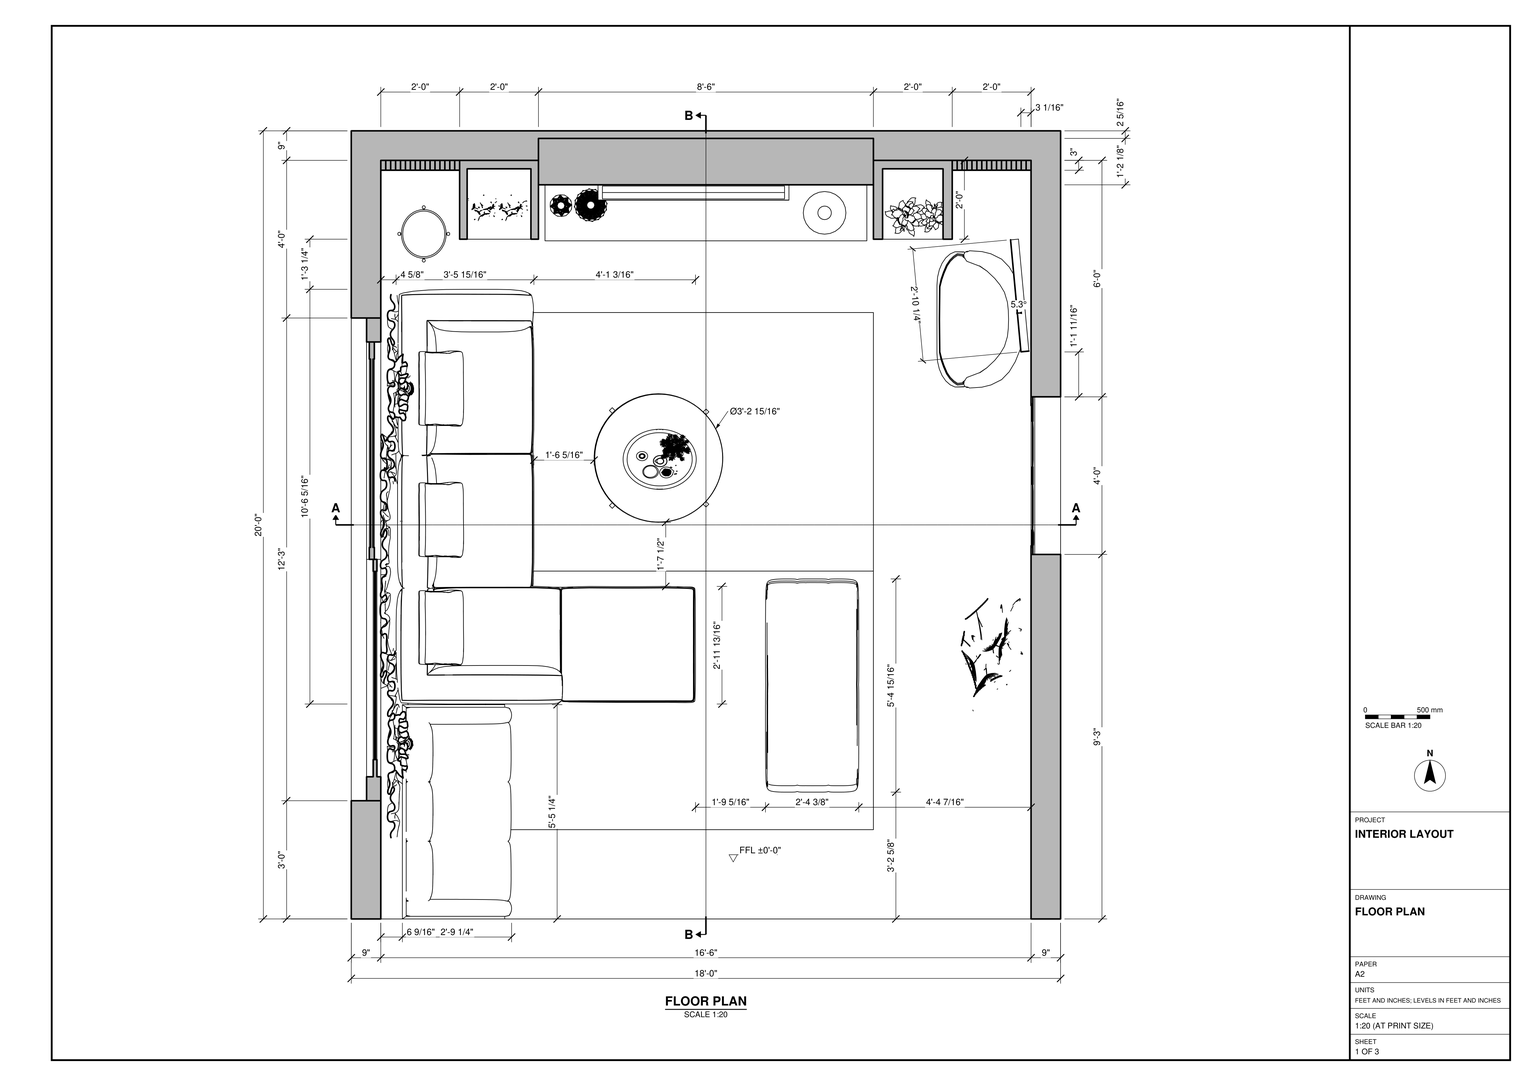
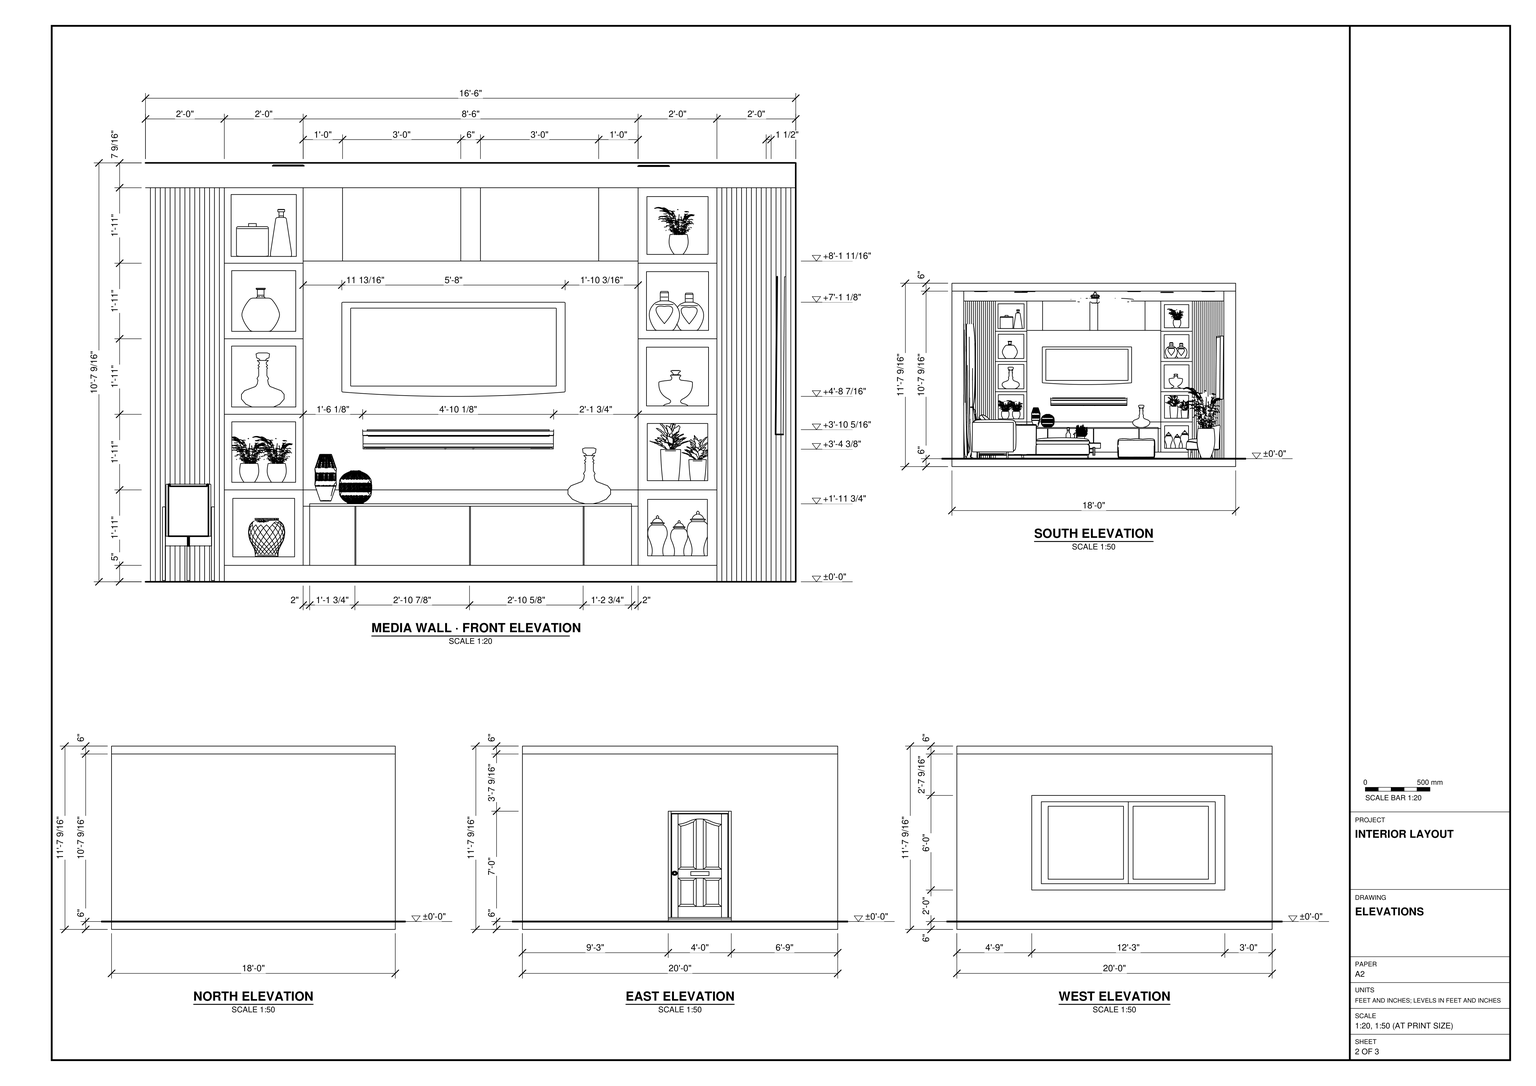
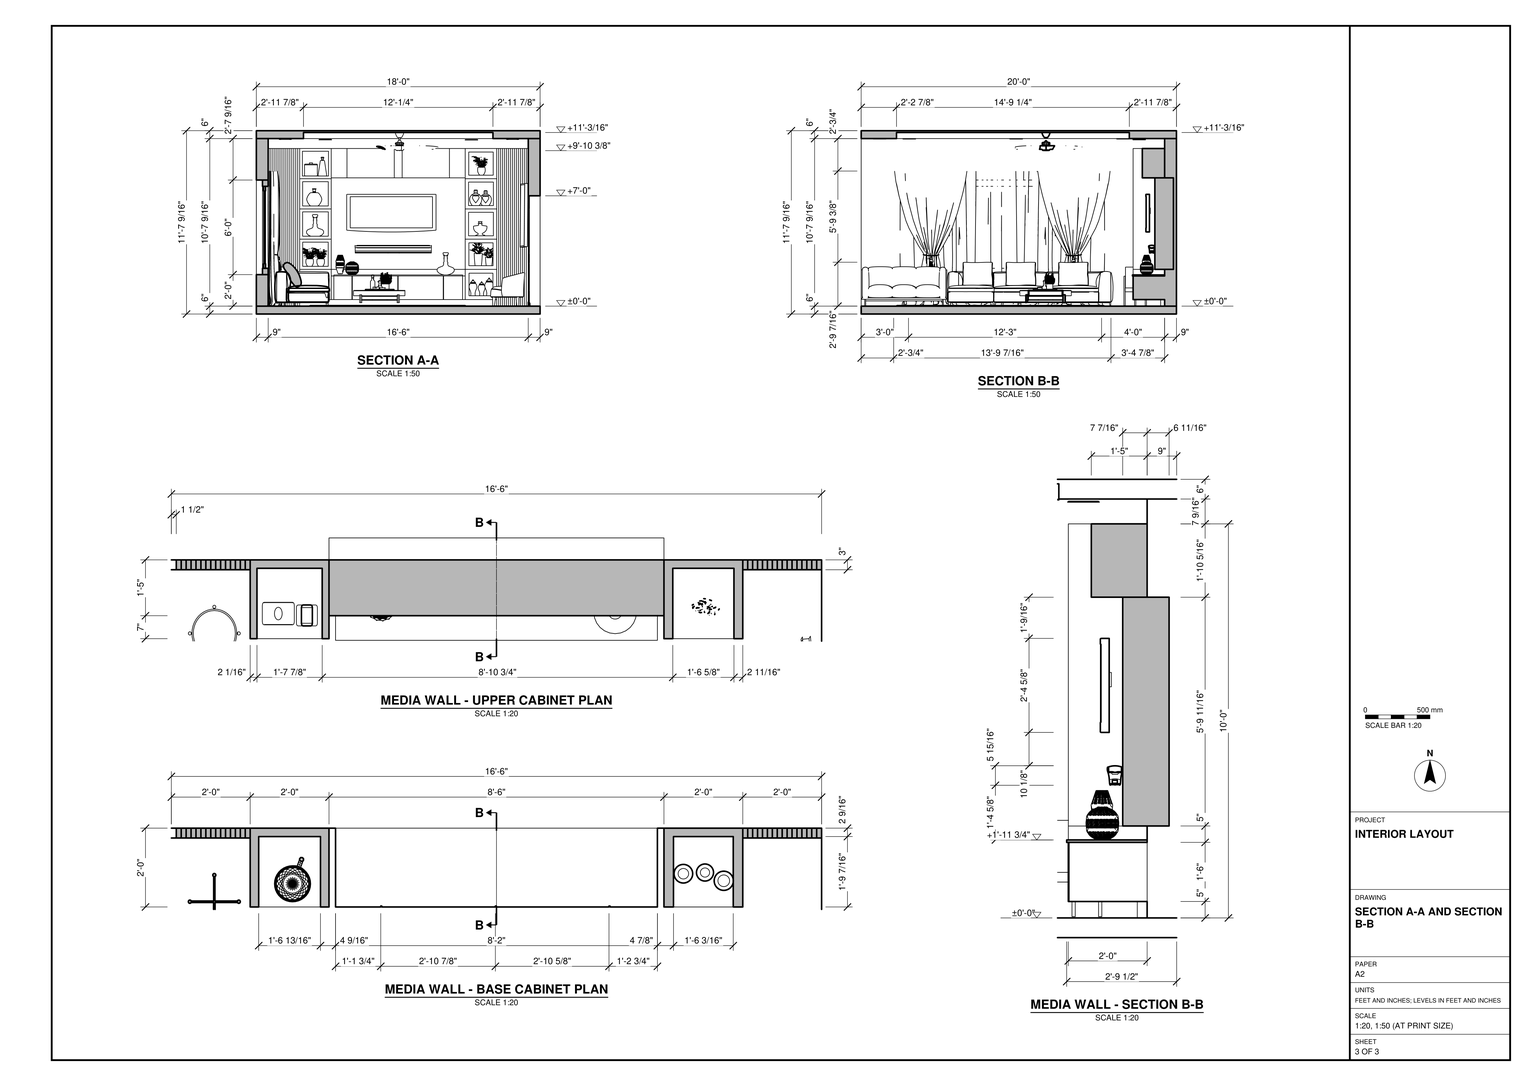
Build the living room in SketchUp from task_files/diagram_01.pdf. Work in feet and inches. The room measures 18'-0" east to west by 20'-0" north to south, with an overall height of 11'-7 9/16". Use ±0'-0" as the finished floor level. Model the 9" walls on the north, east and west sides, leaving the south side open as shown. Include the floor and roof slabs, the stepped ceiling, the framed window and curtains on the west wall, and the door in the east wall.

Fit the media joinery across the north wall. Use the front elevation for the cabinet divisions and shelf spacing, and the cabinet plans and section for the depths, plinth and projections. Place the screen and horizontal speaker between the base and upper cabinets. Flank this bay with open display shelves and finish the outer ends with vertical slats.

Arrange the sectional sofa along the window wall with its chaise extending into the room. Place the round coffee table beside the sectional, the long ottoman east of the chaise, the separate seat at the southwest end and the armchair near the northeast corner. Include the rug beneath the seating area, the ceiling fan and the display objects in the positions shown. Decor and loose items may be any suitable library components, for example from 3D Warehouse.

Keep the walls, slabs and roof, and each furniture or joinery piece, in separate groups or components. Use components for repeated parts. Save one SketchUp model as output_files/furnished_living_room_with_a_built_in_media_wall.skp.

# SketchUp Ruby script. Lengths in inches.
U = 1.inch
M = Sketchup.active_model
def pt(a) = Geom::Point3d.new(a.map { |v| v * U })
def face(e, loops, mat)
  f = e.add_face(loops[0].map { |a| pt(a) })
  loops[1..].each { |l| e.add_face(l.map { |a| pt(a) }).erase! }
  f.material = f.back_material = mat if mat
  f
end
# faces: each face lists its corners as indices into pts; further lists are holes
def faces(e, pts, list, mat = nil) = list.each { |f| face(e, (f[0].is_a?(Array) ? f : [f]).map { |l| l.map { |i| pts[i] } }, mat) }
# xy, xz, yz: faces in a plane at the given z, y or x. An outline is a flat list of corners, or four numbers for a rectangle; further outlines are holes
def ring(l) = l.size == 4 ? [[l[0], l[1]], [l[2], l[1]], [l[2], l[3]], [l[0], l[3]]] : l.each_slice(2).to_a
def flat(e, list, mat, &to3) = list.each { |f| face(e, (f[0].is_a?(Array) ? f : [f]).map { |l| ring(l).map { |u, v| to3.(u, v) } }, mat) }
def xy(e, z, list, mat = nil) = flat(e, list, mat) { |x, y| [x, y, z] }
def xz(e, y, list, mat = nil) = flat(e, list, mat) { |x, z| [x, y, z] }
def yz(e, x, list, mat = nil) = flat(e, list, mat) { |y, z| [x, y, z] }
def lines(e, pts, list) = list.each { |a, b| e.add_line(pt(pts[a]), pt(pts[b])) }
# prism: a flat outline (further loops are holes) pulled along v
def prism(e, loops, v, mat = nil)
  f = face(e, loops, mat); d = Geom::Vector3d.new(v.map { |x| x * U })
  f.pushpull(f.normal.samedirection?(d) ? d.length : -d.length)
end
def box(e, o, s, mat = nil) = prism(e, [[o, [o[0] + s[0], o[1], o[2]], [o[0] + s[0], o[1] + s[1], o[2]], [o[0], o[1] + s[1], o[2]]]], [0, 0, s[2]], mat)
def at(x, y, z, deg = 0) = Geom::Transformation.translation(pt([x, y, z])) * Geom::Transformation.rotation(ORIGIN, Z_AXIS, deg.degrees)
def axes(o, x, y, z) = Geom::Transformation.new([*x, 0, *y, 0, *z, 0, *pt(o).to_a, 1])
def part(name) = M.definitions.add(name)
# library, detail: a bought-in or finely detailed component or shape, given as its bounding box
def library(name, o, s) = part(name).tap { |d| box(d.entities, o, s) }
def detail(e, o, s) = box(e.add_group.entities, o, s)
def put(e, d, t, mat = nil) = e.add_instance(d, t).tap { |i| i.material = mat if mat }
def group(e, t, mat = nil) = e.add_group.tap { |g| g.transformation = t; g.material = mat if mat }.entities
root = M.entities
M.materials.add("CANDLELIGHT BEIGE UC96693").color = [242, 236, 220]
M.materials.add("Translucide ambre1").color = [255, 156, 130]
M.materials["Translucide ambre1"].alpha = 0.5
M.materials.add("Transparence  25").color = [255, 255, 255]
M.materials.add("[Carrera Marble]").color = [207, 207, 207]
M.materials.add("[Color D01]").color = [255, 240, 188]
M.materials.add("[Color D02]").color = [255, 229, 153]
M.materials.add("[Color M08]1").color = [30, 30, 30]
M.materials.add("[Formica Beige]").color = [211, 187, 149]
M.materials.add("[Quartz Light Brown]").color = [242, 230, 205]
M.materials.add("[Translucent_Glass_Safety]").color = [204, 235, 244]
M.materials["[Translucent_Glass_Safety]"].alpha = 0.5
M.materials.add("[Translucent_Glass_Sky_Reflection]").color = [125, 138, 183]
M.materials["[Translucent_Glass_Sky_Reflection]"].alpha = 0.52
M.materials.add("[Wood Bamboo]").color = [198, 132, 75]
M.materials.add("[Wood Floor Light]").color = [204, 176, 127]
M.materials.add("z1").color = [147, 146, 137]
c1 = part("Sliding window")
xy(c1.entities,0,[[0,0,4.33,55.51]])
xy(c1.entities,2.76,[[0,2.76,2,27.76],[3.15,2.76,4.33,27.76],[0,27.76,0.82,52.76],[0.82,27.76,2.36,52.76],[2.36,27.76,4.33,52.76]])
xy(c1.entities,4.72,[[2,4.72,2.4,26.38],[2.76,4.72,3.15,26.38],[0.82,29.13,1.22,50.79],[1.97,29.13,2.36,50.79]])
xy(c1.entities,36.61,[[2,4.72,2.4,26.38],[2.76,4.72,3.15,26.38],[0.82,29.13,1.22,50.79],[1.97,29.13,2.36,50.79]])
xy(c1.entities,38.58,[[0,2.76,2,27.76],[3.15,2.76,4.33,27.76],[0,27.76,0.82,52.76],[0.82,27.76,2.36,52.76],[2.36,27.76,4.33,52.76]])
xy(c1.entities,41.34,[[0,0,4.33,55.51]])
xz(c1.entities,0,[[0,0,4.33,41.34]])
xz(c1.entities,2.76,[[0,2.76,2,38.58],[3.15,2.76,4.33,38.58]])
xz(c1.entities,4.72,[[2,4.72,2.4,36.61],[2.76,4.72,3.15,36.61]])
xz(c1.entities,26.38,[[2,4.72,2.4,36.61],[2.76,4.72,3.15,36.61]])
xz(c1.entities,27.76,[[0.82,2.76,2,38.58],[2,2.76,2.36,38.58],[2.36,2.76,3.15,38.58]])
xz(c1.entities,29.13,[[0.82,4.72,1.22,36.61],[1.97,4.72,2.36,36.61]])
xz(c1.entities,50.79,[[0.82,4.72,1.22,36.61],[1.97,4.72,2.36,36.61]])
xz(c1.entities,52.76,[[0,2.76,0.82,38.58],[0.82,2.76,2.36,38.58],[2.36,2.76,4.33,38.58]])
xz(c1.entities,55.51,[[0,0,4.33,41.34]])
yz(c1.entities,0,[[[0,0,55.51,41.34],[2.76,2.76,52.76,38.58]]])
yz(c1.entities,0.82,[[[27.76,2.76,52.76,38.58],[29.13,4.72,50.79,36.61]]])
yz(c1.entities,1.22,[[29.13,4.72,50.79,36.61]],"[Translucent_Glass_Sky_Reflection]")
yz(c1.entities,1.97,[[29.13,4.72,50.79,36.61]],"[Translucent_Glass_Sky_Reflection]")
yz(c1.entities,2,[[[2.76,2.76,27.76,38.58],[4.72,4.72,26.38,36.61]]])
yz(c1.entities,2.36,[[[27.76,2.76,52.76,38.58],[29.13,4.72,50.79,36.61]]])
yz(c1.entities,2.4,[[4.72,4.72,26.38,36.61]],"[Translucent_Glass_Safety]")
yz(c1.entities,2.76,[[4.72,4.72,26.38,36.61]],"[Translucent_Glass_Safety]")
yz(c1.entities,3.15,[[[2.76,2.76,27.76,38.58],[4.72,4.72,26.38,36.61]]])
yz(c1.entities,4.33,[[[0,0,55.51,41.34],[2.76,2.76,52.76,38.58]]])
c2 = library("door2",[0,0,0],[35.42,7.875,78.74])
c3 = library("michel-club1",[-34.67,-0.85,-0.13],[126.28,91.17,33.41])
c4 = library("BANK+STOEL+MET+RONDE+LEUNING",[-13.09,-13.32,0],[26.18,25.9,25.63])
c5 = library("25984",[-0.01,-37.35,0],[37.87,32.46,16.84])
c6 = part("DDR842RVS01100X")
xy(c6.entities,0,[[-70.87,0,47.24,78.74]])
xy(c6.entities,0.39,[[-70.87,0,47.24,78.74]],"[Quartz Light Brown]")
xz(c6.entities,0,[[-70.87,0,47.24,0.39]])
xz(c6.entities,78.74,[[-70.87,0,47.24,0.39]])
yz(c6.entities,-70.87,[[0,0,78.74,0.39]])
yz(c6.entities,47.24,[[0,0,78.74,0.39]])
c7 = library("Potted plant",[1.65,0,0],[13.63,13.63,20.73])
c8 = library("Group3\#1",[-238.15,54.18,0],[46.4,43.96,56.68])
c9 = library("Untitled",[82.71,28.87,-11.8125],[39.77,1.97,25.2])
c10 = library("Wisdom Sage Series P38m ( On Wall )",[6.24,4.69,38.8125],[7.11,5.95,34.2])
c11 = library("Plant+pots+03",[-13.35,-27.09,0],[26.22,40.73,41.57])
c12 = library("Light+01",[-2.3,-2.42,-0.19],[4.85,4.84,0.19])
c13 = library("Avation+Styled+Ceiling+Fan_JSB",[-19.77,-29.63,-13.8125],[51.59,58.16,13.8125])
c14 = library("Group\#2",[0,0,0],[10.53,165.43,102.59])
c15 = part("Group\#3")
xy(c15.entities,120,[[0,0,1.5,3]])
xz(c15.entities,0,[[0,0,1.5,120]])
yz(c15.entities,1.5,[[0,5,3,120]])
c16 = library("Group\#5",[0,0,0],[112.99,39.26,34.22])
c17 = library("Group\#11",[0,0,0],[33.52,33.48,12.25])
c18 = part("Groupe\#39")
xy(c18.entities,0.1,[[0.39,0.3125,3.55,1.07]],"Translucide ambre1")
xy(c18.entities,3.46,[[0.2,0,3.75,0,3.85,0.03,3.92,0.1,3.94,0.2,3.94,1.18,3.92,1.28,3.85,1.35,3.75,1.38,0.2,1.38,0.1,1.35,0.03,1.28,0,1.18,0,0.2,0.03,0.1,0.1,0.03]])
xz(c18.entities,0,[[0.2,0.2,3.75,3.46]],"Translucide ambre1")
xz(c18.entities,1.38,[[0.2,0.2,3.75,3.46]],"Translucide ambre1")
yz(c18.entities,0,[[0.2,0.2,1.18,3.46]],"Translucide ambre1")
yz(c18.entities,3.94,[[0.2,0.2,1.18,3.46]],"Translucide ambre1")
p = [[0.15,0.11,0.03],[0.11,0.05,0.1],[0.05,0.11,0.1],[0.11,0.15,0.03],[0.2,0.1,0.03],[0.2,0.03,0.1],
  [3.75,0.1,0.03],[3.75,0.03,0.1],[3.8,0.11,0.03],[3.83,0.05,0.1],[3.83,0.15,0.03],[3.9,0.11,0.1],
  [0.03,0.2,0.1],[0.1,0.2,0.03],[0.2,0.2,0],[3.75,0.2,0],[3.85,0.2,0.03],[3.92,0.2,0.1],
  [0.1,1.18,0.03],[0.03,1.18,0.1],[0.2,1.18,0],[0.39,1.07,0.1],[0.39,0.3125,0.1],[3.55,0.3125,0.1],
  [3.55,1.07,0.1],[3.75,1.18,0],[3.85,1.18,0.03],[3.92,1.18,0.1],[0.11,1.33,0.1],[0.15,1.27,0.03],
  [0.11,1.23,0.03],[0.05,1.27,0.1],[0.2,1.28,0.03],[3.75,1.28,0.03],[3.83,1.23,0.03],[3.8,1.27,0.03],
  [3.9,1.27,0.1],[3.83,1.33,0.1],[0.2,1.35,0.1],[3.75,1.35,0.1],[0.1,0.03,0.2],[0.03,0.1,0.2],
  [0.2,0,0.2],[3.75,0,0.2],[3.85,0.03,0.2],[3.92,0.1,0.2],[0,0.2,0.2],[3.94,0.2,0.2],
  [0,1.18,0.2],[3.94,1.18,0.2],[0.03,1.28,0.2],[3.92,1.28,0.2],[0.1,1.35,0.2],[0.2,1.38,0.2],
  [3.75,1.38,0.2],[3.85,1.35,0.2],[0.1,0.03,3.46],[0.03,0.1,3.46],[0.2,0,3.46],[3.75,0,3.46],
  [3.85,0.03,3.46],[3.92,0.1,3.46],[0,0.2,3.46],[3.94,0.2,3.46],[0.03,1.28,3.46],[0,1.18,3.46],
  [3.92,1.28,3.46],[3.94,1.18,3.46],[0.1,1.35,3.46],[3.85,1.35,3.46],[0.2,1.38,3.46],[3.75,1.38,3.46]]
faces(c18.entities,p,[[0,1,2,3],[4,5,1,0],[4,6,7,5],[7,6,8,9],[9,8,10,11],[3,2,12,13],[14,0,3],[14,3,13],
  [14,4,0],[14,15,6,4],[8,15,10],[10,15,16],[6,15,8],[11,10,16,17],[18,13,12,19],[20,14,13,18],
  [20,21,22,14],[14,22,23,15],[24,25,15,23],[15,25,26,16],[16,26,27,17],[25,24,21,20],[28,29,30,31],[31,30,18,19],
  [29,20,30],[30,20,18],[32,20,29],[25,20,32,33],[25,34,26],[25,33,35],[25,35,34],[34,36,27,26],
  [35,37,36,34],[38,32,29,28],[33,32,38,39],[33,39,37,35],[1,40,41,2],[5,42,40,1],[5,7,43,42],[43,7,9,44],
  [44,9,11,45],[2,41,46,12],[45,11,17,47],[19,12,46,48],[17,27,49,47],[50,31,19,48],[36,51,49,27],[52,28,31,50],
  [53,38,28,52],[39,54,55,37],[37,55,51,36],[39,38,53,54],[40,56,57,41],[42,58,56,40],[59,43,44,60],[60,44,45,61],
  [41,57,62,46],[61,45,47,63],[64,50,48,65],[51,66,67,49],[68,52,50,64],[55,69,66,51],[70,53,52,68],[54,71,69,55]],"Translucide ambre1")
c19 = part("Groupe\#53")
prism(c19.entities,[[[0,0.47,0],[0,0.53,0],[0.01,0.59,0],[0.03,0.65,0],[0.06,0.7,0],[0.09,0.75,0],[0.13,0.8,0],[0.17,0.84,0],[0.22,0.87,0],[0.27,0.9,0],[0.33,0.92,0],[0.38,0.9375,0],[0.44,0.95,0],[0.5,0.95,0],[0.5625,0.9375,0],[0.62,0.92,0],[0.68,0.9,0],[0.73,0.87,0],[0.78,0.84,0],[0.82,0.8,0],[0.86,0.75,0],[0.89,0.7,0],[0.91,0.65,0],[0.93,0.59,0],[0.94,0.53,0],[0.95,0.47,0],[0.94,0.41,0],[0.93,0.35,0],[0.91,0.3,0],[0.89,0.24,0],[0.86,0.19,0],[0.82,0.15,0],[0.78,0.11,0],[0.73,0.07,0],[0.68,0.04,0],[0.62,0.02,0],[0.5625,0.01,0],[0.5,0,0],[0.44,0,0],[0.38,0.01,0],[0.33,0.02,0],[0.27,0.04,0],[0.22,0.07,0],[0.17,0.11,0],[0.13,0.15,0],[0.09,0.19,0],[0.06,0.24,0],[0.03,0.3,0],[0.01,0.35,0],[0,0.41,0]]],[0,0,0.38])
c20 = part("Groupe\#24")
xy(c20.entities,0.1,[[0.39,0.3125,3.55,1.07]])
xy(c20.entities,3.66,[[0.2,0.2,3.75,1.18]])
xz(c20.entities,0,[[[0.2,0.2,3.75,3.46],[0.8125,0.8125,3.13,2.85]]])
xz(c20.entities,0,[[0.8125,0.8125,3.13,2.85]],"CANDLELIGHT BEIGE UC96693")
xz(c20.entities,1.38,[[0.2,0.2,3.75,3.46]])
yz(c20.entities,0,[[0.2,0.2,1.18,3.46]])
yz(c20.entities,3.94,[[0.2,0.2,1.18,3.46]])
p = [[0.15,0.11,0.03],[0.11,0.05,0.1],[0.05,0.11,0.1],[0.11,0.15,0.03],[0.2,0.1,0.03],[0.2,0.03,0.1],
  [3.75,0.1,0.03],[3.75,0.03,0.1],[3.8,0.11,0.03],[3.83,0.05,0.1],[3.83,0.15,0.03],[3.9,0.11,0.1],
  [0.03,0.2,0.1],[0.1,0.2,0.03],[0.2,0.2,0],[3.75,0.2,0],[3.85,0.2,0.03],[3.92,0.2,0.1],
  [0.1,1.18,0.03],[0.03,1.18,0.1],[0.2,1.18,0],[0.39,1.07,0.1],[0.39,0.3125,0.1],[3.55,0.3125,0.1],
  [3.55,1.07,0.1],[3.75,1.18,0],[3.85,1.18,0.03],[3.92,1.18,0.1],[0.11,1.33,0.1],[0.15,1.27,0.03],
  [0.11,1.23,0.03],[0.05,1.27,0.1],[0.2,1.28,0.03],[3.75,1.28,0.03],[3.83,1.23,0.03],[3.8,1.27,0.03],
  [3.9,1.27,0.1],[3.83,1.33,0.1],[0.2,1.35,0.1],[3.75,1.35,0.1],[0.1,0.03,0.2],[0.03,0.1,0.2],
  [0.2,0,0.2],[3.75,0,0.2],[3.85,0.03,0.2],[3.92,0.1,0.2],[0,0.2,0.2],[3.94,0.2,0.2],
  [0,1.18,0.2],[3.94,1.18,0.2],[0.03,1.28,0.2],[3.92,1.28,0.2],[0.1,1.35,0.2],[0.2,1.38,0.2],
  [3.75,1.38,0.2],[3.85,1.35,0.2],[0.1,0.03,3.46],[0.03,0.1,3.46],[0.2,0,3.46],[3.75,0,3.46],
  [3.85,0.03,3.46],[3.92,0.1,3.46],[0,0.2,3.46],[3.94,0.2,3.46],[0.03,1.28,3.46],[0,1.18,3.46],
  [3.92,1.28,3.46],[3.94,1.18,3.46],[0.1,1.35,3.46],[3.85,1.35,3.46],[0.2,1.38,3.46],[3.75,1.38,3.46],
  [0.11,0.05,3.5625],[0.05,0.11,3.5625],[0.2,0.03,3.5625],[3.75,0.03,3.5625],[3.83,0.05,3.5625],[3.9,0.11,3.5625],
  [0.03,0.2,3.5625],[3.92,0.2,3.5625],[0.03,1.18,3.5625],[3.92,1.18,3.5625],[0.05,1.27,3.5625],[3.9,1.27,3.5625],
  [0.11,1.33,3.5625],[0.2,1.35,3.5625],[3.75,1.35,3.5625],[3.83,1.33,3.5625],[0.15,0.11,3.64],[0.11,0.15,3.64],
  [0.2,0.1,3.64],[3.75,0.1,3.64],[3.8,0.11,3.64],[3.83,0.15,3.64],[0.1,0.2,3.64],[0.2,0.2,3.66],
  [3.75,0.2,3.66],[3.85,0.2,3.64],[0.1,1.18,3.64],[0.2,1.18,3.66],[3.75,1.18,3.66],[3.85,1.18,3.64],
  [0.15,1.27,3.64],[0.11,1.23,3.64],[0.2,1.28,3.64],[3.75,1.28,3.64],[3.8,1.27,3.64],[3.83,1.23,3.64]]
faces(c20.entities,p,[[0,1,2,3],[4,5,1,0],[4,6,7,5],[7,6,8,9],[9,8,10,11],[3,2,12,13],[14,0,3],[14,3,13],
  [14,4,0],[14,15,6,4],[8,15,10],[10,15,16],[6,15,8],[11,10,16,17],[18,13,12,19],[20,14,13,18],
  [20,21,22,14],[14,22,23,15],[24,25,15,23],[15,25,26,16],[16,26,27,17],[25,24,21,20],[28,29,30,31],[31,30,18,19],
  [29,20,30],[30,20,18],[32,20,29],[25,20,32,33],[25,34,26],[25,33,35],[25,35,34],[34,36,27,26],
  [35,37,36,34],[38,32,29,28],[33,32,38,39],[33,39,37,35],[1,40,41,2],[5,42,40,1],[5,7,43,42],[43,7,9,44],
  [44,9,11,45],[2,41,46,12],[45,11,17,47],[19,12,46,48],[17,27,49,47],[50,31,19,48],[36,51,49,27],[52,28,31,50],
  [53,38,28,52],[39,54,55,37],[37,55,51,36],[39,38,53,54],[40,56,57,41],[42,58,56,40],[59,43,44,60],[60,44,45,61],
  [41,57,62,46],[61,45,47,63],[64,50,48,65],[51,66,67,49],[68,52,50,64],[55,69,66,51],[70,53,52,68],[54,71,69,55],
  [56,72,73,57],[58,74,72,56],[75,74,58,59],[75,59,60,76],[76,60,61,77],[57,73,78,62],[77,61,63,79],[78,80,65,62],
  [81,79,63,67],[82,64,65,80],[66,83,81,67],[84,68,64,82],[85,70,68,84],[71,86,87,69],[69,87,83,66],[85,86,71,70],
  [72,88,89,73],[74,90,88,72],[91,90,74,75],[91,75,76,92],[92,76,77,93],[73,89,94,78],[90,95,88],[88,95,89],
  [89,95,94],[96,95,90,91],[96,91,92],[96,92,93],[96,93,97],[93,77,79,97],[94,98,80,78],[95,99,98,94],
  [100,96,97,101],[101,97,79,81],[102,84,82,103],[103,82,80,98],[99,104,102],[99,102,103],[99,103,98],[99,100,105,104],
  [105,100,106],[106,100,107],[107,100,101],[83,107,101,81],[87,106,107,83],[104,85,84,102],[104,105,86,85],[86,105,106,87]])
c21 = part("Groupe\#77")
put(c21.entities,c19,at(1.5,0.375,3.66),"Transparence  25")
put(c21.entities,c20,axes([0,0,0],[1,0,0],[0,1.23,0],[0,0,1]),"Transparence  25")
c22 = part("Groupe\#128")
put(c22.entities,c18,axes([0.06,0.03,0.05],[0.97,0,0],[0,1.1931,0],[0,0,0.97]),"Translucide ambre1")
put(c22.entities,c21,at(0,0,0))
c23 = library("Group\#20",[0,0,0],[4.2,4.19,4.43])
c24 = library("Group\#21",[0,0,0],[3.96,1.38,4.54])
c25 = library("Group\#24",[0,0,0],[2.58,1.57,5.86])
c26 = library("Group\#25",[0,0,0],[159.9,159.9,209.38])
c27 = library("Group\#30",[0,0,0],[2.89,0.98,3.73])
c28 = library("Group\#203",[0,0,0],[42.29,73.125,63.36])
c29 = library("Group\#213",[0,0,0],[12.8,10.5625,11.04])
c30 = library("Group\#33",[0,0,0],[16.42,7.45,12.07])
c31 = library("Group\#48",[0,0,0],[18.31,18.31,13.72])
xy(root,-6,[[0,0,216,240]],"[Color D02]")
xy(root,0,[[9,0,207,0,207,111,216,111,216,159,207,159,207,231,184.5,231,184.5,228,183,228,183,231,9,231]],"[Color D01]")
xy(root,0,[[0,0,9,0,9,231,207,231,207,159,216,159,216,240,0,240],[207,0,216,111],[183,228,184.5,231]],"[Color D02]")
xy(root,5,[[33,207,57,231],[59,207,59,231,157,231,157,207,142.5625,207,142.5625,207.3,142.26,207.3,142.26,207,107.96,207,107.96,207.3,107.66,207.3,107.66,207,73.0625,207,73.0625,207.3,72.76,207.3,72.76,207],[159,207,183,231]],"[Color D02]")
xy(root,7.59,[[35.59,207,54.41,228.4375]],"[Wood Bamboo]")
xy(root,7.9,[[161.9,207,180.1,228.4375]],"[Wood Bamboo]")
xy(root,23,[[59,206.5,72.76,207],[72.76,206.5,73.0625,207.3],[73.0625,206.5,107.66,207],[107.66,206.5,107.96,207.3],[107.96,206.5,142.26,207],
  [142.26,206.5,142.5625,207.3],[142.5625,206.5,157,207],[59,207,59,231,157,231,157,207,142.5625,207,142.5625,207.3,142.26,207.3,142.26,207,107.96,207,107.96,207.3,107.66,207.3,107.66,207,73.0625,207,73.0625,207.3,72.76,207.3,72.76,207]],"[Color D02]")
xy(root,23.75,[[59,206.5,157,231]],"[Wood Bamboo]")
xy(root,24,[[0,36,9,183]],"[Color D02]")
xy(root,25.1,[[161.9,207,180.1,228.4375]],"[Wood Bamboo]")
xy(root,25.41,[[35.59,207,54.41,228.4375]],"[Wood Bamboo]")
xy(root,28,[[57,223.5625,159,231],[57,231,159,237.6875]],"[Color D02]")
xy(root,30.29,[[35.29,207,54.71,228.4375]],"[Wood Bamboo]")
xy(root,30.79,[[161.79,207,180.21,228.4375]],"[Wood Bamboo]")
xy(root,48.21,[[161.79,207,180.21,228.4375]],"[Wood Bamboo]")
xy(root,48.71,[[35.29,207,54.71,228.4375]])
xy(root,53.23,[[35.23,207,54.77,228.4375]],"[Wood Bamboo]")
xy(root,53.55,[[161.55,207,180.45,228.4375]],"[Wood Bamboo]")
xy(root,71.45,[[161.55,207,180.45,228.4375]],"[Wood Bamboo]")
xy(root,71.77,[[35.23,207,54.77,228.4375]],"[Wood Bamboo]")
xy(root,76.25,[[35.25,207,54.75,228.4375]],"[Wood Bamboo]")
xy(root,76.55,[[161.55,207,180.45,228.4375]],"[Wood Bamboo]")
xy(root,84,[[207,111,216,159]],"[Color D02]")
xy(root,94.45,[[161.55,207,180.45,228.4375]],"[Wood Bamboo]")
xy(root,94.75,[[35.25,207,54.75,228.4375]],"[Wood Bamboo]")
xy(root,96,[[0,36,9,183]],"[Color D02]")
xy(root,97.67,[[57,214,159,223.5625],[57,223.5625,159,231],[57,231,159,237.6875]],"[Color D02]")
xy(root,99.07,[[35.07,207,54.93,228.4375]],"[Wood Bamboo]")
xy(root,99.6875,[[161.6875,207,180.3125,228.4375]],"[Wood Bamboo]")
xy(root,117.3125,[[161.6875,207,180.3125,228.4375]],"[Wood Bamboo]")
xy(root,117.93,[[35.07,207,54.93,228.4375]],"[Wood Bamboo]")
xy(root,120,[[57,214,159,231]],"[Color D01]")
xy(root,120,[[33,207,57,231],[159,207,183,231]],"[Wood Bamboo]")
xy(root,127.5625,[[0,0,0,240,216,240,216,0,207,0,207,231,9,231,9,0],[[9,0,207,231],[35.89,26.89,180.11,204.11]]],"[Color D01]")
xy(root,132.1875,[[35.89,26.89,180.11,204.11]],"[Color D01]")
xy(root,133.5625,[[0,0,216,240]])
xz(root,0,[[0,127.5625,216,133.5625]])
xz(root,0,[[0,0,9,127.5625],[207,0,216,127.5625]],"[Color D01]")
xz(root,0,[[0,-6,216,0]],"[Color D02]")
xz(root,26.89,[[35.89,127.5625,180.11,132.1875]])
xz(root,36,[[0,24,9,96]],"[Color D02]")
xz(root,111,[[207,0,216,84]],"[Color D02]")
xz(root,159,[[207,0,216,84]],"[Color D02]")
xz(root,183,[[0,24,9,96]],"[Color D02]")
xz(root,204.11,[[35.89,127.5625,180.11,132.1875]],"[Color D01]")
xz(root,206.5,[[59,23,157,23.75]],"[Wood Bamboo]")
xz(root,207,[[59,5,72.76,23],[73.0625,5,107.66,23],[107.96,5,142.26,23],[142.5625,5,157,23]],"[Color D01]")
xz(root,207,[[[33,5,57,28],[35.59,7.59,54.41,25.41]],[[159,5,183,28],[161.9,7.9,180.1,25.1]],[[33,28,57,51],[35.29,30.29,54.71,48.71]],[[159,28,183,51],[161.79,30.79,180.21,48.21]],[[33,51,57,74],[35.23,53.23,54.77,71.77]],
  [[159,51,183,74],[161.55,53.55,180.45,71.45]],[[33,74,57,97],[35.25,76.25,54.75,94.75]],[[159,74,183,97],[161.55,76.55,180.45,94.45]],[[33,97,57,120],[35.07,99.07,54.93,117.93]],[[159,97,183,120],[161.6875,99.6875,180.3125,117.3125]]],"[Wood Bamboo]")
xz(root,207.3,[[72.76,5,73.0625,23],[107.66,5,107.96,23],[142.26,5,142.5625,23]],"[Wood Bamboo]")
xz(root,214,[[57,97.67,69,120],[69,97.67,105,120],[105,97.67,111,120],[111,97.67,147,120],[147,97.67,159,120]],"[Color D01]")
xz(root,223.5625,[[57,28,159,97.67]],"[Carrera Marble]")
xz(root,228.4375,[[35.59,7.59,54.41,25.41],[161.9,7.9,180.1,25.1],[35.29,30.29,54.71,48.71],[161.79,30.79,180.21,48.21],[35.23,53.23,54.77,71.77],
  [161.55,53.55,180.45,71.45],[35.25,76.25,54.75,94.75],[161.55,76.55,180.45,94.45],[35.07,99.07,54.93,117.93],[161.6875,99.6875,180.3125,117.3125]],"[Wood Bamboo]")
xz(root,231,[[9,0,183,0,183,5,33,5,33,120,183,120,183,0,207,0,207,127.5625,9,127.5625],[57,23,59,23,59,23.75,157,23.75,157,23,159,23,159,28,57,28]],"[Color D01]")
xz(root,231,[[33,5,57,120],[57,5,59,23],[157,5,159,23],[159,5,183,120],[59,23,157,23.75],
  [57,97.67,159,120]],"[Color D02]")
xz(root,237.6875,[[57,28,159,97.67]],"[Color D02]")
xz(root,240,[[0,127.5625,216,133.5625]])
xz(root,240,[[0,-6,216,0],[0,0,216,127.5625]],"[Color D02]")
yz(root,0,[[0,127.5625,240,133.5625]])
yz(root,0,[[0,-6,240,0],[[0,0,240,127.5625],[36,24,183,96]]],"[Color D02]")
yz(root,9,[[[0,0,231,127.5625],[36,24,183,96]]],"[Color D01]")
yz(root,33,[[207,5,231,120]],"[Wood Bamboo]")
yz(root,35.07,[[207,99.07,228.4375,117.93]],"[Wood Bamboo]")
yz(root,35.23,[[207,53.23,228.4375,71.77]],"[Wood Bamboo]")
yz(root,35.25,[[207,76.25,228.4375,94.75]],"[Wood Bamboo]")
yz(root,35.29,[[207,30.29,228.4375,48.71]],"[Wood Bamboo]")
yz(root,35.59,[[207,7.59,228.4375,25.41]],"[Wood Bamboo]")
yz(root,35.89,[[26.89,127.5625,204.11,132.1875]],"[Color D01]")
yz(root,54.41,[[207,7.59,228.4375,23],[207,23,228.4375,25.41]],"[Wood Bamboo]")
yz(root,54.71,[[207,30.29,228.4375,48.71]],"[Wood Bamboo]")
yz(root,54.75,[[207,76.25,228.4375,94.75]],"[Wood Bamboo]")
yz(root,54.77,[[207,53.23,228.4375,71.77]],"[Wood Bamboo]")
yz(root,54.93,[[207,99.07,228.4375,117.93]],"[Wood Bamboo]")
yz(root,57,[[223.5625,28,231,97.67],[231,28,237.6875,97.67],[214,97.67,231,120]],"[Color D02]")
yz(root,57,[[207,5,231,23],[207,23,231,28],[207,28,223.5625,28,223.5625,97.67,214,97.67,214,120,207,120]],"[Wood Bamboo]")
yz(root,59,[[207,5,231,23],[206.5,23,231,23.75]],"[Color D02]")
yz(root,72.76,[[207,5,207.3,23]],"[Color D02]")
yz(root,73.0625,[[207,5,207.3,23]],"[Color D02]")
yz(root,107.66,[[207,5,207.3,23]],"[Color D02]")
yz(root,107.96,[[207,5,207.3,23]],"[Color D02]")
yz(root,142.26,[[207,5,207.3,23]],"[Color D02]")
yz(root,142.5625,[[207,5,207.3,23]],"[Color D02]")
yz(root,157,[[207,5,231,23],[206.5,23,231,23.75]],"[Color D02]")
yz(root,159,[[223.5625,28,231,97.67],[231,28,237.6875,97.67],[214,97.67,231,120]],"[Color D02]")
yz(root,159,[[207,5,231,23],[207,23,231,28],[207,28,207,120,214,120,214,97.67,223.5625,97.67,223.5625,28]],"[Wood Bamboo]")
yz(root,161.55,[[207,53.55,228.4375,71.45],[207,76.55,228.4375,94.45]],"[Wood Bamboo]")
yz(root,161.6875,[[207,99.6875,228.4375,117.3125]],"[Wood Bamboo]")
yz(root,161.79,[[207,30.79,228.4375,48.21]],"[Wood Bamboo]")
yz(root,161.9,[[207,7.9,228.4375,23],[207,23,228.4375,25.1]],"[Wood Bamboo]")
yz(root,180.1,[[207,7.9,228.4375,25.1]],"[Wood Bamboo]")
yz(root,180.11,[[26.89,127.5625,204.11,132.1875]],"[Color D01]")
yz(root,180.21,[[207,30.79,228.4375,48.21]],"[Wood Bamboo]")
yz(root,180.3125,[[207,99.6875,228.4375,117.3125]],"[Wood Bamboo]")
yz(root,180.45,[[207,53.55,228.4375,71.45],[207,76.55,228.4375,94.45]],"[Wood Bamboo]")
yz(root,183,[[228,0,231,5],[228,5,231,120]],"[Color D02]")
yz(root,183,[[207,5,228,120]],"[Wood Bamboo]")
yz(root,184.5,[[228,0,231,5]],"[Color D02]")
yz(root,207,[[0,0,0,127.5625,231,127.5625,231,0,159,0,159,84,111,84,111,0]],"[Color D01]")
yz(root,216,[[0,127.5625,240,133.5625]])
yz(root,216,[[0,0,111,0,111,84,159,84,159,0,240,0,240,127.5625,0,127.5625]],"[Color D01]")
yz(root,216,[[0,-6,240,0]],"[Color D02]")
put(root,c1,axes([4.67,36,24],[1,0,0],[0,2.64809,0],[0,0,1.74171]))
put(root,c2,axes([208.125,159,0],[0,-1.35518,0],[-0.143,0,0],[0,0,1.0668]))
put(root,c3,at(103.97,100.12,0.13,90),"[Formica Beige]")
put(root,c4,axes([190.93,182.58,0],[0,1.59651,0],[-1,0,0],[0,0,1]))
put(root,c5,axes([126.14,113.32,0],[0.75,0,0],[0,2,0],[0,0,0.91]))
put(root,c6,at(111.75,27.19,0),"[Quartz Light Brown]")
put(root,c6,at(111.75,105.93,0))
put(root,c7,axes([12.26,200.02,0.39],[1.16,0,0],[0,1.26,0],[0,0,1.4148]))
put(root,c8,axes([405.99,-33.5625,0],[1,0,0],[0,1.58,0],[0,0,1.0089]))
put(root,c9,axes([-72.65,167.38,69.89],[1.71,0,0],[0,1.71,0],[0,0,1.13763]))
put(root,c10,axes([199.26,214.75,51.01],[0,0.66,0],[0,0,-1],[-1.7,0,0]))
put(root,c8,axes([262.71,196.68,99.6875],[0.42974,0,0],[0,0.2664,0],[0,0,0.2664]))
put(root,c8,axes([131.96,196.58,29.96],[0.42974,0,0],[0,0.2664,0],[0,0,0.2664]))
put(root,c8,axes([140.33,196.58,29.96],[0.42974,0,0],[0,0.2664,0],[0,0,0.2664]))
put(root,c11,axes([168.91,213.94,28],[0,0.52,0],[-0.52,0,0],[0,0,0.52]))
put(root,c12,axes([21.79,199.36,127.5625],[2,0,0],[0,2,0],[0,0,2]))
put(root,c12,axes([194.85,199.36,127.5625],[2,0,0],[0,2,0],[0,0,2]))
put(root,c12,axes([194.85,117.98,127.5625],[2,0,0],[0,2,0],[0,0,2]))
put(root,c12,axes([21.79,117.98,127.5625],[2,0,0],[0,2,0],[0,0,2]))
put(root,c12,axes([194.85,36.61,127.5625],[2,0,0],[0,2,0],[0,0,2]))
put(root,c12,axes([21.79,36.61,127.5625],[2,0,0],[0,2,0],[0,0,2]))
put(root,c12,axes([52.24,211.62,126.95],[2,0,0],[0,2,0],[0,0,2]))
put(root,c12,axes([163.49,212.37,126.83],[2,0,0],[0,2,0],[0,0,2]))
put(root,c12,axes([58.18,14.05,127.5625],[2,0,0],[0,2,0],[0,0,2]))
put(root,c12,axes([138.43,14.05,127.5625],[2,0,0],[0,2,0],[0,0,2]))
put(root,c13,at(109,140.66,132.1875))
put(root,c14,at(8.8,24.72,0.23))
put(root,c15,at(183,228,0),"[Wood Floor Light]")
put(root,c15,at(184.5,228,0),"[Wood Floor Light]")
put(root,c15,at(186,228,0),"[Wood Floor Light]")
put(root,c15,at(187.5,228,0),"[Wood Floor Light]")
put(root,c15,at(189,228,0),"[Wood Floor Light]")
put(root,c15,at(190.5,228,0),"[Wood Floor Light]")
put(root,c15,at(192,228,0),"[Wood Floor Light]")
put(root,c15,at(193.5,228,0),"[Wood Floor Light]")
put(root,c15,at(195,228,0),"[Wood Floor Light]")
put(root,c15,at(196.5,228,0),"[Wood Floor Light]")
put(root,c15,at(198,228,0),"[Wood Floor Light]")
put(root,c15,at(199.5,228,0),"[Wood Floor Light]")
put(root,c15,at(201,228,0),"[Wood Floor Light]")
put(root,c15,at(202.5,228,0),"[Wood Floor Light]")
put(root,c15,at(204,228,0),"[Wood Floor Light]")
put(root,c15,at(205.5,228,0),"[Wood Floor Light]")
put(root,c15,at(24,228,0),"[Wood Floor Light]")
put(root,c15,at(25.5,228,0),"[Wood Floor Light]")
put(root,c15,at(30,228,0),"[Wood Floor Light]")
put(root,c15,at(27,228,0),"[Wood Floor Light]")
put(root,c15,at(31.5,228,0),"[Wood Floor Light]")
put(root,c15,at(22.5,228,0),"[Wood Floor Light]")
put(root,c15,at(28.5,228,0),"[Wood Floor Light]")
put(root,c15,at(9,228,0),"[Wood Floor Light]")
put(root,c15,at(21,228,0),"[Wood Floor Light]")
put(root,c15,at(10.5,228,0),"[Wood Floor Light]")
put(root,c15,at(15,228,0),"[Wood Floor Light]")
put(root,c15,at(12,228,0),"[Wood Floor Light]")
put(root,c15,at(13.5,228,0),"[Wood Floor Light]")
put(root,c15,at(16.5,228,0),"[Wood Floor Light]")
put(root,c15,at(18,228,0),"[Wood Floor Light]")
put(root,c15,at(19.5,228,0),"[Wood Floor Light]")
put(root,c16,axes([48.82,0,0],[0,0.5775,0],[-0.847,0,0],[0,0,0.8778]))
put(root,c17,axes([73.94,120.79,2.625],[1.17,0,0],[0,1.17,0],[0,0,0.76752]))
put(root,c22,axes([36.7,211.22,99.11],[2.46906,0,0],[0,4.04926,0],[0,0,2.46906]))
put(root,c23,axes([165.3,215.875,53.55],[2.44,0,0],[0,2.44,0],[0,0,2.44]))
put(root,c24,axes([38.35,213.94,76.25],[2.8944,0,0],[0,4.94942,0],[0,0,2.8944]))
put(root,c25,axes([47.08,210.89,98.93],[2.46906,0,0],[0,4.04926,0],[0,0,2.46906]))
put(root,c26,axes([38.23,212.41,52.6875],[0.08122,0,0],[0,0.08122,0],[0,0,0.08122]))
put(root,c27,axes([162.4,215.26,76.55],[3.1842,0,0],[0,3.1842,0],[0,0,3.1842]))
put(root,c27,axes([170.15,215.4,76.55],[3.045,0,0],[0,3.045,0],[0,0,3.045]))
put(root,c28,axes([60.56,222.4,23.75],[0,-0.23786,0],[0.23786,0,0],[0,0,0.23786]))
put(root,c29,axes([52.28,209.53,7.73],[-0.17491,1.03411,0],[-1.03411,-0.17491,0],[0,0,1.0488]))
put(root,c26,axes([137.64,208.53,23.75],[0.08122,0,0],[0,0.08122,0],[0,0,0.08122]))
put(root,c30,axes([161.9375,211.68,7.9],[1.1305,0,0],[0,1.1305,0],[0,0,1.1305]))
put(root,c31,axes([82.78,130.82,12.04],[1.21624,0,0],[0,1,0],[0,0,1]))
g1 = group(root,at(206.75,173.65,93.375))
p = [[-6.01,33.15,-48.52],[-2.84,-0.97,-48.01],[-0.41,-0.75,-48.04],[-3.59,33.37,-48.54],[-2.43,-0.23,0.02],[-5.6,33.89,-0.48],
  [-5.53,33.07,-1.29],[-5.93,32.34,-47.6875],[-2.91,-0.14,-47.21],[-2.51,0.58,-0.81],[0,0,0],[-3.17,34.12,-0.5]]
faces(g1,p,[[0,1,2,3],[1,4,10,2],[7,6,9,8]],"z1")
faces(g1,p,[[[4,1,0,5],[6,7,8,9]]],"[Color M08]1")
lines(g1,p,[[10,11],[11,3]])
